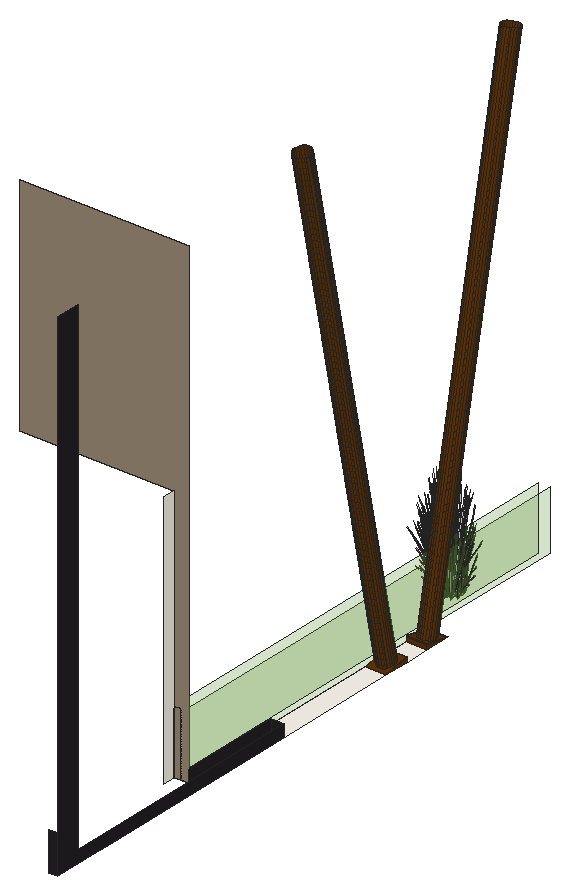
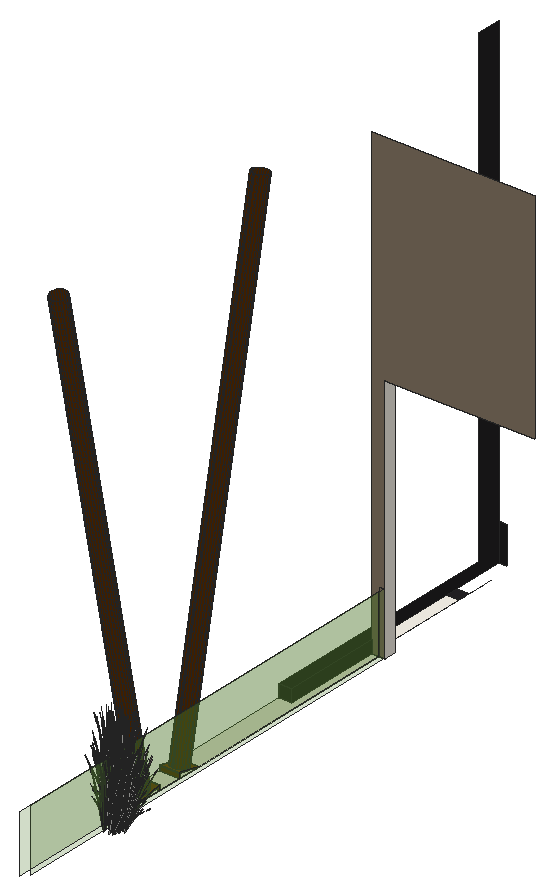
# SketchUp Ruby script. Lengths in inches.
U = 1.inch
M = Sketchup.active_model
def pt(a) = Geom::Point3d.new(a.map { |v| v * U })
def face(e, loops, mat)
  f = e.add_face(loops[0].map { |a| pt(a) })
  loops[1..].each { |l| e.add_face(l.map { |a| pt(a) }).erase! }
  f.material = f.back_material = mat if mat
  f
end
# faces: each face lists its corners as indices into pts; further lists are holes
def faces(e, pts, list, mat = nil) = list.each { |f| face(e, (f[0].is_a?(Array) ? f : [f]).map { |l| l.map { |i| pts[i] } }, mat) }
# xy, xz, yz: faces in a plane at the given z, y or x. An outline is a flat list of corners, or four numbers for a rectangle; further outlines are holes
def ring(l) = l.size == 4 ? [[l[0], l[1]], [l[2], l[1]], [l[2], l[3]], [l[0], l[3]]] : l.each_slice(2).to_a
def flat(e, list, mat, &to3) = list.each { |f| face(e, (f[0].is_a?(Array) ? f : [f]).map { |l| ring(l).map { |u, v| to3.(u, v) } }, mat) }
def xy(e, z, list, mat = nil) = flat(e, list, mat) { |x, y| [x, y, z] }
def xz(e, y, list, mat = nil) = flat(e, list, mat) { |x, z| [x, y, z] }
def yz(e, x, list, mat = nil) = flat(e, list, mat) { |y, z| [x, y, z] }
def lines(e, pts, list) = list.each { |a, b| e.add_line(pt(pts[a]), pt(pts[b])) }
# prism: a flat outline (further loops are holes) pulled along v
def prism(e, loops, v, mat = nil)
  f = face(e, loops, mat); d = Geom::Vector3d.new(v.map { |x| x * U })
  f.pushpull(f.normal.samedirection?(d) ? d.length : -d.length)
end
def box(e, o, s, mat = nil) = prism(e, [[o, [o[0] + s[0], o[1], o[2]], [o[0] + s[0], o[1] + s[1], o[2]], [o[0], o[1] + s[1], o[2]]]], [0, 0, s[2]], mat)
def at(x, y, z, deg = 0) = Geom::Transformation.translation(pt([x, y, z])) * Geom::Transformation.rotation(ORIGIN, Z_AXIS, deg.degrees)
def axes(o, x, y, z) = Geom::Transformation.new([*x, 0, *y, 0, *z, 0, *pt(o).to_a, 1])
def part(name) = M.definitions.add(name)
# library, detail: a bought-in or finely detailed component or shape, given as its bounding box
def library(name, o, s) = part(name).tap { |d| box(d.entities, o, s) }
def detail(e, o, s) = box(e.add_group.entities, o, s)
def put(e, d, t, mat = nil) = e.add_instance(d, t).tap { |i| i.material = mat if mat }
def group(e, t, mat = nil) = e.add_group.tap { |g| g.transformation = t; g.material = mat if mat }.entities
root = M.entities
M.materials.add("C01_Vanilla_Cream").color = [255, 251, 241]
M.materials.add("C08_Toffee_Ember").color = [102, 51, 0]
M.materials.add("Glass_Basic_01").color = [119, 186, 61]
M.materials["Glass_Basic_01"].alpha = 0.25
M.materials.add("LightPink_Translucent").color = [144, 107, 117]
M.materials["LightPink_Translucent"].alpha = 0.75
M.materials.add("Marble_07_1K").color = [36, 34, 36]
M.materials.add("Plaster_02_1K").color = [157, 140, 119]
c1 = part("blade")
p = [[2.15,0.21,22],[0,0.17,0],[0.09,0.45,0],[2.18,0.31,22],[2.29,0.31,22],[0.38,0.45,0],
  [2.48,0.24,33],[2.49,0.24,33],[2.48,0.22,33]]
faces(c1.entities,p,[[0,1,2,3],[4,5,2,3],[6,3,4,7],[8,0,3,6]])
c2 = part("seeds")
p = [[0.3,-0.1,1.38],[-0.01,-0.03,1.59],[-0.01,-0.03,0.03],[0.14,-0.07,-0.07],[0.29,-0.03,3],[0.15,0.01,3.11]]
faces(c2.entities,p,[[0,1,2,3],[1,0,4,5]],"LightPink_Translucent")
c3 = part("blade with seeds")
put(c3.entities,c1,at(0,0,0))
put(c3.entities,c2,axes([2.4,0.25,30.99],[1.5799,-0.05474,1.17369],[-0.12525,1.92788,0.29478],[-0.07173,-0.02425,1.56792]))
xy(root,390,[[700,91.21,706,192],[696.41,144,700,144,700,192,706,192,706,252,696.41,252],[696.41,252,706,264],[696.41,264,706,276],[696.41,276,701.21,288],
  [701.21,276,706,288]],"C01_Vanilla_Cream")
xy(root,390,[[700,85.38,706,91.21]],"Marble_07_1K")
xz(root,60,[[702,390,706,408]],"Marble_07_1K")
xz(root,144,[[696.41,390,696.41,420,693.41,420,693.41,510,621.41,510,621.41,615,700,615,700,390],[693.41,390,696.41,420]],"Plaster_02_1K")
xz(root,192,[[700,390,706,396]],"Marble_07_1K")
xz(root,264,[[696.41,390,706,392],[696.41,392,706,392.5]],"C08_Toffee_Ember")
xz(root,276,[[696.41,390,706,392],[696.41,392,706,392.5]],"C08_Toffee_Ember")
yz(root,693.41,[[138,390,144,510]],"C01_Vanilla_Cream")
yz(root,693.41,[[144,390,357,420]],"Glass_Basic_01")
yz(root,696.41,[[144,390,252,390,264,392.5,264,390,276,390,276,392.5,288,390,360,390,360,418,144,418],[252,390,264,390,264,392],[252,390,264,392,264,392.5],[276,390,288,390,276,392],[288,390,276,392.5,276,392]],"Glass_Basic_01")
yz(root,700,[[144,390,192,396]],"Marble_07_1K")
yz(root,706,[[252,390,264,390,264,392],[252,390,264,392,264,392.5],[276,390,288,390,276,392],[288,390,276,392.5,276,392]],"C08_Toffee_Ember")
yz(root,706,[[60,390,192,390,192,396,72,396,72,624,60,624]],"Marble_07_1K")
p = [[706,252,390],[706,258,391],[696.41,258,391],[696.41,252,390],[706,264,392.5],[696.41,264,392.5],
  [696.41,258,391.25],[697.24,258,391.25],[697.27,258.72,391.4],[697.6,259.6875,391.6],[698.17,260.54,391.78],[698.94,261.23,391.92],
  [699.87,261.69,392.02],[700.89,261.9,392.0625],[701.21,261.89,392.06],[701.9375,261.85,392.05],[702.93,261.53,391.99],[703.81,260.98,391.87],
  [704.5,260.22,391.71],[704.98,259.31,391.52],[705.19,258.31,391.3125],[705.18,258,391.25],[705.14,257.28,391.1],[704.82,256.3125,390.9],
  [704.25,255.46,390.72],[703.47,254.77,390.58],[702.54,254.31,390.48],[701.52,254.1,390.4375],[701.21,254.11,390.44],[700.48,254.15,390.45],
  [699.48,254.47,390.51],[698.61,255.02,390.63],[697.91,255.78,390.79],[697.4375,256.69,390.98],[697.22,257.69,391.1875],[700.17,285.78,390.46],
  [701.21,285.92,390.43],[702.24,285.78,390.46],[703.21,285.39,390.54],[704.04,284.77,390.67],[704.67,283.96,390.84],[705.07,283.01,391.04],
  [705.21,282,391.25],[706,282,391.25],[706,288,390],[701.21,288,390],[696.41,288,390],[696.41,282,391.25],
  [697.21,282,391.25],[697.34,283.01,391.04],[697.74,283.96,390.84],[698.38,284.77,390.67],[699.21,285.39,390.54],[696.41,282,391],
  [701.21,282,391],[706,282,391],[700.48,205.24,625.23],[699.48,205.55,625.3],[701.21,205.2,625.22],[701.52,205.18,625.22],
  [702.54,205.39,625.26],[700.17,334.7,625.25],[701.21,334.83,625.22],[702.24,334.7,625.25],[703.47,205.86,625.36],[698.61,206.11,625.41],
  [698.38,333.68,625.46],[699.21,334.3,625.33],[703.21,334.3,625.33],[704.04,333.68,625.46],[704.25,206.54,625.5],[697.91,206.87,625.57],
  [704.82,207.4,625.68],[697.74,332.87,625.625],[704.67,332.87,625.625],[697.4375,207.78,625.76],[697.34,331.93,625.82],[705.07,331.93,625.82],
  [705.14,208.37,625.88],[697.22,208.78,625.97],[696.41,264,392],[706,264,392],[701.21,264,392],[701.21,276,392],
  [696.41,276,392],[706,276,392],[697.21,330.91,626.03],[705.21,330.91,626.03],[705.18,209.09,626.03],[697.24,209.09,626.03],
  [697.27,209.8,626.18],[705.19,209.39,626.1],[696.41,276,392.5],[706,276,392.5],[705.07,280.99,391.46],[704.67,280.04,391.66],
  [704.04,279.23,391.83],[703.21,278.61,391.96],[702.24,278.22,392.04],[701.21,278.08,392.07],[700.17,278.22,392.04],[699.21,278.61,391.96],
  [698.38,279.23,391.83],[697.74,280.04,391.66],[697.34,280.99,391.46],[697.34,329.9,626.24],[705.07,329.9,626.24],[704.98,210.39,626.31],
  [697.6,210.77,626.39],[704.5,211.3,626.5],[697.74,328.96,626.44],[704.67,328.96,626.44],[698.17,211.63,626.5625],[703.81,212.0625,626.65],
  [698.38,328.14,626.61],[704.04,328.14,626.61],[698.94,212.31,626.71],[699.21,327.52,626.74],[703.21,327.52,626.74],[702.93,212.62,626.77],
  [699.87,212.78,626.8],[701.9375,212.9375,626.84],[700.89,212.99,626.85],[701.21,327,626.85],[700.17,327.13,626.82],[702.24,327.13,626.82],
  [701.21,212.97,626.84],[700,144,390],[700,72,390],[693.41,144,390]]
faces(root,p,[[0,1,2,3],[46,53,54,45],[45,54,55,44],[80,2,1,81,82],[83,54,53,84],[85,55,54,83]],"C01_Vanilla_Cream")
faces(root,p,[[3,0,4,5,6,7,8,9,10,11,12,13,14,15,16,17,18,19,20,21,22,23,24,25,26,27,28,29,30,31,32,33,34,7,6],[35,36,37,38,39,40,41,42,43,44,45,46,47,48,49,50,51,52],[30,29,56,57],[29,28,58,56],[28,27,59,58],[27,26,60,59],[36,35,61,62],[37,36,62,63],
  [26,25,64,60],[31,30,57,65],[52,51,66,67],[39,38,68,69],[35,52,67,61],[38,37,63,68],[25,24,70,64],[32,31,65,71],
  [24,23,72,70],[51,50,73,66],[40,39,69,74],[33,32,71,75],[50,49,76,73],[41,40,74,77],[23,22,78,72],[34,33,75,79],
  [49,48,86,76],[42,41,77,87],[22,21,88,78],[7,34,79,89],[8,7,89,90],[21,20,91,88],[47,92,93,43,42,94,95,96,97,98,99,100,101,102,103,104,48],[48,104,105,86],
  [94,42,87,106],[20,19,107,91],[9,8,90,108],[19,18,109,107],[104,103,110,105],[95,94,106,111],[10,9,108,112],[18,17,113,109],
  [103,102,114,110],[96,95,111,115],[11,10,112,116],[102,101,117,114],[97,96,115,118],[17,16,119,113],[12,11,116,120],[16,15,121,119],
  [13,12,120,122],[100,99,123,124],[99,98,125,123],[101,100,124,117],[98,97,118,125],[15,14,126,121],[14,13,122,126]],"C08_Toffee_Ember")
lines(root,p,[[127,128],[127,129]])
put(root,c3,axes([686.9,308.77,393.22],[0.14872,0.18332,1.42242],[-0.6872,0.15433,0.11501],[-0.15531,-0.28779,0.60807]))
put(root,c3,axes([688.03,307.56,393.91],[-0.09951,-0.08005,1.45204],[-0.66407,0.05075,-0.22964],[-0.10598,-0.19148,0.11645]))
put(root,c3,axes([689.57,308.51,392.15],[-0.18493,0.11557,1.18691],[-0.55384,-0.20228,-0.25526],[0.10266,-0.25157,0.50747]))
put(root,c3,axes([688.73,308.91,394.13],[-0.31051,-0.46426,-0.58968],[0.63919,-0.25873,0.07116],[-0.07261,-0.22432,0.83415]))
put(root,c3,axes([686.71,308.29,392.15],[-0.0394,0.18678,1.18691],[-0.57594,0.15636,-0.25526],[-0.13463,-0.24142,0.50747]))
put(root,c3,axes([688.2,307.88,391.24],[-0.10912,0.02057,1.46364],[-0.60346,-0.23156,-0.2236],[0.01013,-0.19315,0.24931]))
put(root,c3,axes([690.02,309.37,394.13],[0.01693,-0.52814,-0.58968],[0.71285,0.03547,0.07116],[0.07523,-0.22375,0.83415]))
put(root,c3,axes([691.02,308.54,393.91],[-0.00628,-0.11364,1.45204],[-0.53042,-0.32843,-0.22964],[0.08201,-0.19909,0.11645]))
put(root,c3,axes([688.79,308.52,393.76],[0.19614,-0.43908,-0.29394],[0.57222,0.12807,0.37948],[-0.05247,-0.17678,0.72609]))
put(root,c3,axes([689.22,309.1,393.22],[-0.12114,0.19625,1.42242],[-0.50818,-0.40613,0.11501],[0.22925,-0.25313,0.60807]))
put(root,c3,axes([690.875,308.13,393.91],[-0.06607,0.04361,1.47228],[-0.64734,-0.14714,-0.13912],[-0.02343,-0.19032,0.26054]))
put(root,c3,axes([688.5,308.82,393.89],[-0.63954,-0.14313,-0.42412],[0.21921,-0.49074,-0.32852],[-0.05864,-0.19758,0.81151]))
put(root,c3,axes([688.89,307.59,392.3],[0.08346,0.33295,0.95334],[-0.46298,-0.1844,0.70045],[0.04982,-0.17048,0.20998]))
put(root,c3,axes([689.88,309.19,393.89],[-0.46573,-0.38364,-0.42412],[0.49199,-0.33598,-0.32852],[0.07086,-0.19492,0.81151]))
put(root,c3,axes([687.35,307.3,393.91],[-0.01214,0.06844,1.47228],[-0.59861,0.24837,-0.13912],[-0.17615,-0.12696,0.26054]))
put(root,c3,axes([687.22,308.51,394.23],[0.72473,-0.14676,0.44623],[0.12578,0.57568,0.36794],[-0.17045,-0.16967,0.92337]))
put(root,c3,axes([688.86,308.62,393.93],[0.64106,0.14927,0.39842],[-0.21921,0.49074,0.32852],[-0.03852,-0.19299,0.82444]))
put(root,c3,axes([689.05,308.79,394.18],[-0.63664,0.26583,-0.10093],[-0.31286,-0.47181,-0.56021],[-0.084,-0.19882,0.85122]))
put(root,c3,axes([690.37,309.39,394.18],[-0.71502,-0.02829,-0.10093],[0.01954,-0.53563,-0.56021],[0.04967,-0.20629,0.85122]))
put(root,c3,axes([690.32,309.05,393.76],[0.4402,-0.30062,-0.29394],[0.41671,0.34326,0.37948],[0.0634,-0.1744,0.72609]))
put(root,c3,axes([686.51,307.99,392.3],[0.33937,0.19872,0.95334],[-0.49424,0.11946,0.70045],[-0.10575,-0.15273,0.20998]))
put(root,c3,axes([689.03,308.58,393.93],[0.47939,-0.19405,0.05337],[0.23464,0.35385,0.42015],[-0.0463,-0.15598,0.64067]))
put(root,c3,axes([687.33,309.04,394.13],[-0.55475,-0.27598,-0.58968],[0.39425,-0.48361,0.07116],[-0.20099,-0.16478,0.83415]))
put(root,c3,axes([687.14,308.68,393.76],[-0.10048,-0.4599,-0.29394],[0.5744,-0.12144,0.37948],[-0.15428,-0.13179,0.72609]))
put(root,c3,axes([687.39,308.64,393.93],[0.29569,-0.36271,0.05337],[0.42107,0.21117,0.42015],[-0.13613,-0.11629,0.64067]))
put(root,c3,axes([686.24,308.59,391.24],[-0.06302,0.07522,1.46364],[-0.63686,0.16217,-0.2236],[-0.15385,-0.14752,0.24931]))
put(root,c3,axes([687.3,310.66,391.74],[-0.26718,-0.5855,-0.57963],[0.76964,-0.21087,-0.15213],[-0.02953,-0.19827,1.27944]))
put(root,c3,axes([685.9,309.35,393.22],[0.24166,0.09837,1.42242],[-0.50011,0.41269,0.11501],[-0.3117,-0.18617,0.60807]))
put(root,c3,axes([690.87,308.87,391.24],[-0.09738,-0.04498,1.46364],[-0.25012,-0.50252,-0.2236],[0.16873,-0.13637,0.24931]))
put(root,c3,axes([688.85,308.98,394.19],[-0.19614,0.43908,0.29394],[-0.57222,-0.12807,-0.37948],[-0.05247,-0.17678,0.72609]))
put(root,c3,axes([687.07,309.06,393.89],[-0.64198,0.13573,-0.42412],[-0.1123,-0.514,-0.32852],[-0.17243,-0.1473,0.81151]))
put(root,c3,axes([690.32,309.16,393.93],[0.46327,0.38957,0.39842],[-0.49199,0.33598,0.32852],[0.08546,-0.18277,0.82444]))
put(root,c3,axes([687.52,308.6,394.51],[-0.4342,0.54737,-0.11304],[-0.6288,-0.31535,-0.62743],[-0.21858,-0.15465,0.95337]))
put(root,c3,axes([690.49,309.2,393.93],[0.53464,0.0266,0.05337],[-0.01466,0.40172,0.42015],[0.05594,-0.15388,0.64067]))
put(root,c3,axes([690.09,309.47,394.19],[-0.4402,0.30062,0.29394],[-0.41671,-0.34326,-0.37948],[0.0634,-0.1744,0.72609]))
put(root,c3,axes([690.86,310.28,394.13],[0.33983,-0.45051,-0.58968],[0.59551,0.32017,0.07116],[0.20291,-0.16322,0.83415]))
put(root,c3,axes([687.19,308.97,391.97],[-0.40676,-0.57214,0],[0.68052,-0.31907,-0.42834],[0.15499,-0.07267,1.3588]))
put(root,c3,axes([690.85,310.07,393.89],[-0.16713,-0.52135,-0.42412],[0.63294,-0.0912,-0.32852],[0.18138,-0.14003,0.81151]))
put(root,c3,axes([688.08,308.28,391.77],[-0.44958,0.32756,-0.03231],[-0.41194,-0.35875,-0.14649],[-0.029,-0.10165,0.48318]))
put(root,c3,axes([685.86,308.44,393.91],[-0.13998,-0.00403,1.45204],[-0.44565,0.40302,-0.22964],[-0.23779,-0.08235,0.11645]))
put(root,c3,axes([691.15,310.45,394.18],[-0.60181,-0.31483,-0.10093],[0.34671,-0.45593,-0.56021],[0.17003,-0.15849,0.85122]))
put(root,c3,axes([688.66,312.17,392.76],[0.56221,0.23024,1.25546],[-0.55078,0.49601,0.49647],[-0.2467,-0.29398,1.05249]))
put(root,c3,axes([687.48,309.05,394.19],[0.10048,0.4599,0.29394],[-0.5744,0.12144,-0.37948],[-0.15428,-0.13179,0.72609]))
put(root,c3,axes([685.72,310.57,391.67],[0,-0.57097,-0.4121],[0.72788,0,0],[0,-0.13004,1.30728]))
put(root,c3,axes([687.74,308.88,391.67],[0.60889,-0.28548,-0.4121],[0.36394,0.51192,0],[0.13868,-0.06502,1.30728]))
put(root,c3,axes([691.36,309.87,392.15],[-0.23242,-0.01691,1.18691],[-0.23811,-0.45367,-0.25526],[0.28553,-0.12834,0.50747]))
put(root,c3,axes([685.76,309.35,394.23],[0.53728,-0.42137,0.44623],[0.46337,0.44748,0.36794],[-0.25207,-0.07773,0.92337]))
put(root,c3,axes([692.63,310.31,393.91],[-0.08498,-0.00434,1.47228],[-0.35287,-0.46464,-0.13912],[0.14171,-0.15278,0.26054]))
put(root,c3,axes([688.47,310.05,391.71],[0.43821,-0.42916,-0.51753],[0.54436,0.38915,-0.13583],[0.1756,-0.10706,1.14236]))
put(root,c3,axes([691.625,309.04,392.3],[-0.2167,0.29065,0.95334],[-0.18626,-0.3905,0.70045],[0.17898,-0.09785,0.20998]))
put(root,c3,axes([691.31,310.13,393.76],[0.56631,-0.0816,-0.29394],[0.14954,0.46647,0.37948],[0.16229,-0.12529,0.72609]))
put(root,c3,axes([686,309.35,393.93],[0.03276,-0.43418,0.05337],[0.49468,0.0119,0.42015],[-0.18949,-0.04543,0.64067]))
put(root,c3,axes([687.7,310.81,391.83],[0.31565,-0.51449,-0.37133],[0.65588,0.24761,0.17871],[0,-0.1186,1.19224]))
put(root,c3,axes([685.8125,309.49,393.76],[-0.37017,-0.35748,-0.29394],[0.42268,-0.3384,0.37948],[-0.21476,-0.05149,0.72609]))
put(root,c3,axes([687.99,310.55,392.21],[-0.07581,-0.65151,-0.24149],[0.7896,-0.03939,-0.41502],[0.13904,-0.08678,1.32557]))
put(root,c3,axes([686.03,310.59,391.68],[0.45414,-0.35624,-0.25712],[0.45414,0.35624,0.25712],[0,-0.11474,1.15348]))
put(root,c3,axes([685.85,308.88,391.77],[-0.18768,0.46622,-0.03231],[-0.57763,-0.14342,-0.14649],[-0.0877,-0.07626,0.48318]))
put(root,c3,axes([690.85,310.4,394.19],[-0.56631,0.0816,0.29394],[-0.14954,-0.46647,-0.37948],[0.16229,-0.12529,0.72609]))
put(root,c3,axes([687.625,311.23,392.21],[-0.73268,-0.27244,-0.24149],[0.35279,-0.57501,-0.41502],[-0.02303,-0.14118,1.32557]))
put(root,c3,axes([685.54,311.01,391.97],[-0.81352,0,0],[0,-0.63814,-0.42834],[0,-0.14534,1.3588]))
put(root,c3,axes([687.89,309.11,391.68],[0.60696,0.14127,-0.25712],[-0.15283,0.49751,0.25712],[0.12236,-0.05737,1.15348]))
put(root,c3,axes([691.37,310.33,393.93],[0.44663,0.24013,0.05337],[-0.26003,0.34195,0.42015],[0.14319,-0.11055,0.64067]))
put(root,c3,axes([691.24,310.23,393.93],[0.16135,0.52549,0.39842],[-0.63294,0.0912,0.32852],[0.18654,-0.12359,0.82444]))
put(root,c3,axes([692.95,310.86,393.91],[0.09028,-0.08697,1.45204],[-0.11555,-0.53348,-0.22964],[0.22652,-0.10115,0.11645]))
put(root,c3,axes([686.17,310.84,391.93],[-0.60515,0.48003,0.25528],[-0.60552,-0.47498,-0.30288],[-0.02113,-0.13632,1.36855]))
put(root,c3,axes([685.32,308.78,393.91],[0.04823,0.05698,1.47228],[-0.23252,0.51221,-0.13912],[-0.23548,0.00371,0.26054]))
put(root,c3,axes([688.09,311.0625,392.02],[0.73304,0.27674,0.19974],[-0.35279,0.57501,0.41502],[0,-0.13255,1.3325]))
put(root,c3,axes([687.81,311.84,392.02],[0.17244,-0.67657,-0.19446],[0.81759,0.11793,0.42555],[-0.14286,-0.09343,1.29846]))
put(root,c3,axes([688.07,314.13,393.22],[0.14872,0.18332,1.42242],[-0.6872,0.15433,0.11501],[-0.15531,-0.28779,0.60807]))
put(root,c3,axes([685.99,309.84,393.89],[-0.47241,0.37822,-0.42412],[-0.41372,-0.39954,-0.32852],[-0.24002,-0.05755,0.81151]))
put(root,c3,axes([686.34,309.67,394.19],[0.37017,0.35748,0.29394],[-0.42268,0.3384,-0.37948],[-0.21476,-0.05149,0.72609]))
put(root,c3,axes([689.2,312.92,393.91],[-0.09951,-0.08005,1.45204],[-0.66407,0.05075,-0.22964],[-0.10598,-0.19148,0.11645]))
put(root,c3,axes([684.92,310.34,392.3],[0.41536,-0.04086,0.95334],[-0.26347,0.35999,0.70045],[-0.20525,-0.054,0.20998]))
put(root,c3,axes([690.74,313.87,392.15],[-0.18493,0.11557,1.18691],[-0.55384,-0.20228,-0.25526],[0.10266,-0.25157,0.50747]))
put(root,c3,axes([689.9,314.27,394.13],[-0.31051,-0.46426,-0.58968],[0.63919,-0.25873,0.07116],[-0.07261,-0.22432,0.83415]))
put(root,c3,axes([687.86,310.68,392.26],[-0.70648,0.03525,0.37133],[-0.06389,-0.58508,-0.17871],[0.12647,-0.0593,1.19224]))
put(root,c3,axes([686.23,309.45,394.18],[-0.03484,0.58066,-0.10093],[-0.65957,-0.01587,-0.56021],[-0.25402,-0.04034,0.85122]))
put(root,c3,axes([686.03,311.1,392.06],[0,0.57097,0.4121],[-0.72788,0,0],[0,-0.13004,1.30728]))
put(root,c3,axes([687.88,313.65,392.15],[-0.0394,0.18678,1.18691],[-0.57594,0.15636,-0.25526],[-0.13463,-0.24142,0.50747]))
put(root,c3,axes([691.17,311.67,394.18],[-0.32734,-0.51701,-0.10093],[0.58097,-0.25407,-0.56021],[0.24483,-0.06821,0.85122]))
put(root,c3,axes([691.14,311.23,393.89],[0.17625,-0.51936,-0.42412],[0.60429,0.17802,-0.32852],[0.2433,-0.04762,0.81151]))
put(root,c3,axes([690.1875,309.12,391.97],[0.40676,-0.57214,0],[0.68052,0.31907,-0.42834],[0.15499,0.07267,1.3588]))
put(root,c3,axes([689.37,313.24,391.24],[-0.10912,0.02057,1.46364],[-0.60346,-0.23156,-0.2236],[0.01013,-0.19315,0.24931]))
put(root,c3,axes([687.75,311.5625,391.83],[-0.39083,-0.47924,-0.37133],[0.59199,-0.33747,0.17871],[-0.12647,-0.0593,1.19224]))
put(root,c3,axes([687.83,310.89,391.96],[0.28286,0.63846,0.37976],[-0.80821,0.22202,0.14902],[0.00988,-0.11732,1.31851]))
put(root,c3,axes([691.79,311.38,391.65],[-0.41902,0.06852,1.17514],[-0.0667,-0.54541,0.06726],[0.29348,-0.08255,0.6687]))
put(root,c3,axes([692.55,310.89,391.875],[-0.40335,-0.3651,-0.05385],[0.44175,-0.33453,-0.24415],[0.12517,-0.02355,0.8053]))
put(root,c3,axes([691.19,314.72,394.13],[0.01693,-0.52814,-0.58968],[0.71285,0.03547,0.07116],[0.07523,-0.22375,0.83415]))
put(root,c3,axes([687.69,311.39,392.26],[-0.31565,0.51449,0.37133],[-0.65588,-0.24761,-0.17871],[0,-0.1186,1.19224]))
put(root,c3,axes([688.85,310.94,391.83],[0,-0.66065,0],[0.81352,0,0],[0,0,1.48949]))
put(root,c3,axes([692.1875,313.9,393.91],[-0.00628,-0.11364,1.45204],[-0.53042,-0.32843,-0.22964],[0.08201,-0.19909,0.11645]))
put(root,c3,axes([689.96,313.875,393.76],[0.19614,-0.43908,-0.29394],[0.57222,0.12807,0.37948],[-0.05247,-0.17678,0.72609]))
put(root,c3,axes([690.39,314.46,393.22],[-0.12114,0.19625,1.42242],[-0.50818,-0.40613,0.11501],[0.22925,-0.25313,0.60807]))
put(root,c3,axes([689.84,309.41,392.06],[-0.60889,-0.28548,0.4121],[0.36394,-0.51192,0],[0.13868,0.06502,1.30728]))
put(root,c3,axes([692.05,313.49,393.91],[-0.06607,0.04361,1.47228],[-0.64734,-0.14714,-0.13912],[-0.02343,-0.19032,0.26054]))
put(root,c3,axes([691.03,311.42,394.13],[0.57168,-0.25217,-0.58968],[0.3186,0.51908,0.07116],[0.27622,-0.05897,0.83415]))
put(root,c3,axes([687.4,311.75,391.71],[-0.67676,-0.09361,-0.51753],[0.14281,-0.57742,-0.13583],[-0.20196,-0.06997,1.14236]))
put(root,c3,axes([688.46,310.53,391.96],[-0.53943,0.51816,0.37976],[-0.64086,-0.4574,0.14902],[0.13005,-0.05171,1.31851]))
put(root,c3,axes([689.67,314.18,393.89],[-0.63954,-0.14313,-0.42412],[0.21921,-0.49074,-0.32852],[-0.05864,-0.19758,0.81151]))
put(root,c3,axes([690.0625,312.95,392.3],[0.08346,0.33295,0.95334],[-0.46298,-0.1844,0.70045],[0.04982,-0.17048,0.20998]))
put(root,c3,axes([689.05,311.45,391.91],[-0.60515,-0.49144,-0.05089],[0.60552,-0.49174,0],[-0.02113,-0.01716,1.45724]))
put(root,c3,axes([691.05,314.55,393.89],[-0.46573,-0.38364,-0.42412],[0.49199,-0.33598,-0.32852],[0.07086,-0.19492,0.81151]))
put(root,c3,axes([687.53,309.67,392.05],[-0.18794,0.56744,0.14643],[-0.68774,-0.16058,0.29122],[0.1188,-0.00276,1.33138]))
put(root,c3,axes([690.94,311.52,394.19],[-0.54068,-0.15928,0.29394],[0.1577,-0.46469,-0.37948],[0.21769,-0.04261,0.72609]))
put(root,c3,axes([688.52,312.65,393.91],[-0.01214,0.06844,1.47228],[-0.59861,0.24837,-0.13912],[-0.17615,-0.12696,0.26054]))
put(root,c3,axes([685.28,310.67,393.93],[0.18381,-0.5206,0.39842],[0.60429,0.17802,0.32852],[-0.23764,0.03129,0.82444]))
put(root,c3,axes([687.24,310.13,391.32],[-0.64037,0.22859,1.07011],[-0.20382,-0.65589,0.4158],[0.39323,0.01091,1.21713]))
put(root,c3,axes([688.96,310.3,392.17],[0.12551,-0.50956,0.12018],[0.6132,0.08845,-0.34318],[0.1116,0.05232,1.05198]))
put(root,c3,axes([685.24,310.53,393.93],[-0.23895,-0.38931,0.05337],[0.43573,-0.19055,0.42015],[-0.19208,0.0376,0.64067]))
put(root,c3,axes([687.9,311.51,391.96],[0.82229,0.1203,0.37976],[-0.16734,0.67942,0.14902],[-0.12017,-0.06561,1.31851]))
put(root,c3,axes([692.24,311.02,391.24],[-0.034,-0.08668,1.46364],[0.23582,-0.50706,-0.2236],[0.23788,-0.00729,0.24931]))
put(root,c3,axes([688.39,313.87,394.23],[0.72473,-0.14676,0.44623],[0.12578,0.57568,0.36794],[-0.17045,-0.16967,0.92337]))
put(root,c3,axes([685.22,310.93,391.24],[0.0165,0.08998,1.46364],[-0.33262,0.46992,-0.2236],[-0.23626,-0.02369,0.24931]))
put(root,c3,axes([688.7,310.4375,392.26],[-0.39083,-0.47924,0.37133],[0.59199,-0.33747,-0.17871],[0.12647,0.0593,1.19224]))
put(root,c3,axes([690.03,313.98,393.93],[0.64106,0.14927,0.39842],[-0.21921,0.49074,0.32852],[-0.03852,-0.19299,0.82444]))
put(root,c3,axes([690.22,314.15,394.18],[-0.63664,0.26583,-0.10093],[-0.31286,-0.47181,-0.56021],[-0.084,-0.19882,0.85122]))
put(root,c3,axes([686.68,312.63,391.68],[-0.15283,-0.49751,-0.25712],[0.60696,-0.14127,0.25712],[-0.12236,-0.05737,1.15348]))
put(root,c3,axes([691.54,314.75,394.18],[-0.71502,-0.02829,-0.10093],[0.01954,-0.53563,-0.56021],[0.04967,-0.20629,0.85122]))
put(root,c3,axes([691.49,314.41,393.76],[0.4402,-0.30062,-0.29394],[0.41671,0.34326,0.37948],[0.0634,-0.1744,0.72609]))
put(root,c3,axes([687.68,313.35,392.3],[0.33937,0.19872,0.95334],[-0.49424,0.11946,0.70045],[-0.10575,-0.15273,0.20998]))
put(root,c3,axes([690.2,313.94,393.93],[0.47939,-0.19405,0.05337],[0.23464,0.35385,0.42015],[-0.0463,-0.15598,0.64067]))
put(root,c3,axes([688.5,314.4,394.13],[-0.55475,-0.27598,-0.58968],[0.39425,-0.48361,0.07116],[-0.20099,-0.16478,0.83415]))
put(root,c3,axes([688.31,314.04,393.76],[-0.10048,-0.4599,-0.29394],[0.5744,-0.12144,0.37948],[-0.15428,-0.13179,0.72609]))
put(root,c3,axes([687.46,312.6,392.05],[0.6991,-0.15154,0.14643],[0.17263,0.56398,0.29122],[-0.06235,-0.08217,1.33138]))
put(root,c3,axes([688.9,310.47,392.21],[0.65687,-0.37907,-0.24149],[0.43681,0.53562,-0.41502],[0.16207,0.0544,1.32557]))
put(root,c3,axes([691.51,311.47,393.76],[0.54068,0.15928,-0.29394],[-0.1577,0.46469,0.37948],[0.21769,-0.04261,0.72609]))
put(root,c3,axes([686.51,312.84,391.67],[-0.60889,-0.28548,-0.4121],[0.36394,-0.51192,0],[-0.13868,-0.06502,1.30728]))
put(root,c3,axes([690.56,309.46,391.67],[0.60889,0.28548,-0.4121],[-0.36394,0.51192,0],[0.13868,0.06502,1.30728]))
put(root,c3,axes([685.16,310.73,393.76],[-0.54068,-0.15928,-0.29394],[0.1577,-0.46469,0.37948],[-0.21769,0.04261,0.72609]))
put(root,c3,axes([689.4,311.09,391.83],[0.72788,0,0],[0,0.59111,0],[0,0,1.48078]))
put(root,c3,axes([688.17,311.83,392.21],[-0.65687,0.37907,-0.24149],[-0.43681,-0.53562,-0.41502],[-0.16207,-0.0544,1.32557]))
put(root,c3,axes([689.61,309.7,392.05],[-0.6991,0.15154,0.14643],[-0.17263,-0.56398,0.29122],[0.06235,0.08217,1.33138]))
put(root,c3,axes([688.56,313.99,393.93],[0.29569,-0.36271,0.05337],[0.42107,0.21117,0.42015],[-0.13613,-0.11629,0.64067]))
put(root,c3,axes([687.41,313.95,391.24],[-0.06302,0.07522,1.46364],[-0.63686,0.16217,-0.2236],[-0.15385,-0.14752,0.24931]))
put(root,c3,axes([690.04,310.89,393.22],[-0.26985,0.01293,1.42242],[0.17902,-0.56047,0.11501],[0.38456,0.03467,0.60807]))
put(root,c3,axes([690.39,309.67,391.68],[0.15283,0.49751,-0.25712],[-0.60696,0.14127,0.25712],[0.12236,0.05737,1.15348]))
put(root,c3,axes([688.47,316.01,391.74],[-0.26718,-0.5855,-0.57963],[0.76964,-0.21087,-0.15213],[-0.02953,-0.19827,1.27944]))
put(root,c3,axes([687.07,314.7,393.22],[0.24166,0.09837,1.42242],[-0.50011,0.41269,0.11501],[-0.3117,-0.18617,0.60807]))
put(root,c3,axes([691.43,311.66,393.93],[0.23895,0.38931,0.05337],[-0.43573,0.19055,0.42015],[0.19208,-0.0376,0.64067]))
put(root,c3,axes([692.04,314.22,391.24],[-0.09738,-0.04498,1.46364],[-0.25012,-0.50252,-0.2236],[0.16873,-0.13637,0.24931]))
put(root,c3,axes([689.17,310.79,391.98],[-0.82229,-0.1203,0.40835],[0.16734,-0.67942,0.16024],[0.12017,0.06561,1.41775]))
put(root,c3,axes([691.39,311.53,393.93],[-0.18381,0.5206,0.39842],[-0.60429,-0.17802,0.32852],[0.23764,-0.03129,0.82444]))
put(root,c3,axes([688.51,312.47,391.83],[-0.21227,-0.49226,0],[0.60616,-0.17239,0],[0,0,1.28128]))
put(root,c3,axes([690.02,314.34,394.19],[-0.19614,0.43908,0.29394],[-0.57222,-0.12807,-0.37948],[-0.05247,-0.17678,0.72609]))
put(root,c3,axes([688.11,312,392.17],[-0.12551,0.50956,0.12018],[-0.6132,-0.08845,-0.34318],[-0.1116,-0.05232,1.05198]))
put(root,c3,axes([685.73,310.68,394.19],[0.54068,0.15928,0.29394],[-0.1577,0.46469,-0.37948],[-0.21769,0.04261,0.72609]))
put(root,c3,axes([688.24,314.41,393.89],[-0.64198,0.13573,-0.42412],[-0.1123,-0.514,-0.32852],[-0.17243,-0.1473,0.81151]))
put(root,c3,axes([689.3,312.4,391.8125],[0.68303,-0.19373,-0.15934],[0.24001,0.55805,0.00007],[0.07539,-0.02141,1.44335]))
put(root,c3,axes([691.49,314.52,393.93],[0.46327,0.38957,0.39842],[-0.49199,0.33598,0.32852],[0.08546,-0.18277,0.82444]))
put(root,c3,axes([688.69,313.96,394.51],[-0.4342,0.54737,-0.11304],[-0.6288,-0.31535,-0.62743],[-0.21858,-0.15465,0.95337]))
put(root,c3,axes([689.54,312.63,392.05],[0.18794,-0.56744,0.14643],[0.68774,0.16058,0.29122],[-0.1188,0.00276,1.33138]))
put(root,c3,axes([691.66,314.56,393.93],[0.53464,0.0266,0.05337],[-0.01466,0.40172,0.42015],[0.05594,-0.15388,0.64067]))
put(root,c3,axes([689.39,311.34,391.84],[0.45414,0.3688,0],[-0.45414,0.3688,0],[0,0,1.40491]))
put(root,c3,axes([690.62,311.18,392.05],[-0.51116,-0.4159,0.14643],[0.51512,-0.4034,0.29122],[-0.05645,0.08494,1.33138]))
put(root,c3,axes([691.26,314.83,394.19],[-0.4402,0.30062,0.29394],[-0.41671,-0.34326,-0.37948],[0.0634,-0.1744,0.72609]))
put(root,c3,axes([689.67,310.55,391.71],[0.67676,0.09361,-0.51753],[-0.14281,0.57742,-0.13583],[0.20196,0.06997,1.14236]))
put(root,c3,axes([692.66,311.5625,392.3],[-0.40197,0.09426,0.95334],[0.18921,-0.38956,0.70045],[0.21325,0.02666,0.20998]))
put(root,c3,axes([692.03,315.64,394.13],[0.33983,-0.45051,-0.58968],[0.59551,0.32017,0.07116],[0.20291,-0.16322,0.83415]))
put(root,c3,axes([688.36,314.33,391.97],[-0.40676,-0.57214,0],[0.68052,-0.31907,-0.42834],[0.15499,-0.07267,1.3588]))
put(root,c3,axes([692.02,315.43,393.89],[-0.16713,-0.52135,-0.42412],[0.63294,-0.0912,-0.32852],[0.18138,-0.14003,0.81151]))
put(root,c3,axes([689.25,313.64,391.77],[-0.44958,0.32756,-0.03231],[-0.41194,-0.35875,-0.14649],[-0.029,-0.10165,0.48318]))
put(root,c3,axes([688.36,312.6875,391.82],[-0.65588,-0.25634,0],[0.31565,-0.53263,0],[0,0,1.35047]))
put(root,c3,axes([688.91,312.01,392.05],[-0.63528,-0.45956,-0.20909],[0.53456,-0.51604,0.45758],[-0.17107,0.05376,1.39619]))
put(root,c3,axes([687.23,312.89,392.06],[0.60889,0.28548,0.4121],[-0.36394,0.51192,0],[-0.13868,-0.06502,1.30728]))
put(root,c3,axes([689.38,310.91,392.26],[0.31565,-0.51449,0.37133],[0.65588,0.24761,-0.17871],[0,0.1186,1.19224]))
put(root,c3,axes([687.03,313.8,393.91],[-0.13998,-0.00403,1.45204],[-0.44565,0.40302,-0.22964],[-0.23779,-0.08235,0.11645]))
put(root,c3,axes([692.32,315.8,394.18],[-0.60181,-0.31483,-0.10093],[0.34671,-0.45593,-0.56021],[0.17003,-0.15849,0.85122]))
put(root,c3,axes([692.47,313.21,393.91],[-0.05883,-0.04999,1.47228],[0.12868,-0.53581,-0.13912],[0.23172,-0.03423,0.26054]))
put(root,c3,axes([689.26,311.21,391.9],[0,0.66033,-0.04679],[-0.81352,0,0],[0,0.02075,1.48875]))
put(root,c3,axes([685.53,310.96,393.89],[-0.17625,0.51936,-0.42412],[-0.60429,-0.17802,-0.32852],[-0.2433,0.04762,0.81151]))
put(root,c3,axes([685.5,310.52,394.18],[0.32734,0.51701,-0.10093],[-0.58097,0.25407,-0.56021],[-0.24483,0.06821,0.85122]))
put(root,c3,axes([689.32,310.74,391.83],[0.39083,0.47924,-0.37133],[-0.59199,0.33747,0.17871],[0.12647,0.0593,1.19224]))
put(root,c3,axes([691.96,312.76,393.26],[-0.12452,-0.47997,-0.02898],[0.58854,-0.11034,-0.1314],[0.1229,0.03043,0.43341]))
put(root,c3,axes([686.88,313.19,391.97],[-0.40676,0.57214,0],[-0.68052,-0.31907,-0.42834],[-0.15499,-0.07267,1.3588]))
put(root,c3,axes([689.83,317.52,392.76],[0.56221,0.23024,1.25546],[-0.55078,0.49601,0.49647],[-0.2467,-0.29398,1.05249]))
put(root,c3,axes([690.44,312.75,394.18],[0.03484,-0.58066,-0.10093],[0.65957,0.01587,-0.56021],[0.25402,0.04034,0.85122]))
put(root,c3,axes([688.65,314.41,394.19],[0.10048,0.4599,0.29394],[-0.5744,0.12144,-0.37948],[-0.15428,-0.13179,0.72609]))
put(root,c3,axes([691.04,311.2,392.06],[0,-0.57097,0.4121],[0.72788,0,0],[0,0.13004,1.30728]))
put(root,c3,axes([686.89,315.93,391.67],[0,-0.57097,-0.4121],[0.72788,0,0],[0,-0.13004,1.30728]))
put(root,c3,axes([688.91,314.24,391.67],[0.60889,-0.28548,-0.4121],[0.36394,0.51192,0],[0.13868,-0.06502,1.30728]))
put(root,c3,axes([689.21,311.625,392.26],[0.70648,-0.03525,0.37133],[0.06389,0.58508,-0.17871],[-0.12647,0.0593,1.19224]))
put(root,c3,axes([689.65,311.03,392.17],[0.60616,-0.16651,0.12018],[0.21227,0.47548,-0.34318],[0,0.10465,1.05198]))
put(root,c3,axes([692.53,315.23,392.15],[-0.23242,-0.01691,1.18691],[-0.23811,-0.45367,-0.25526],[0.28553,-0.12834,0.50747]))
